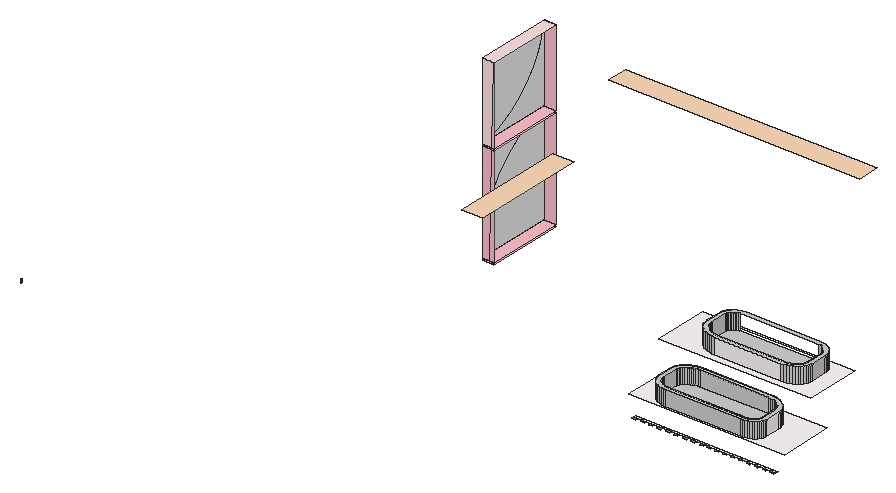
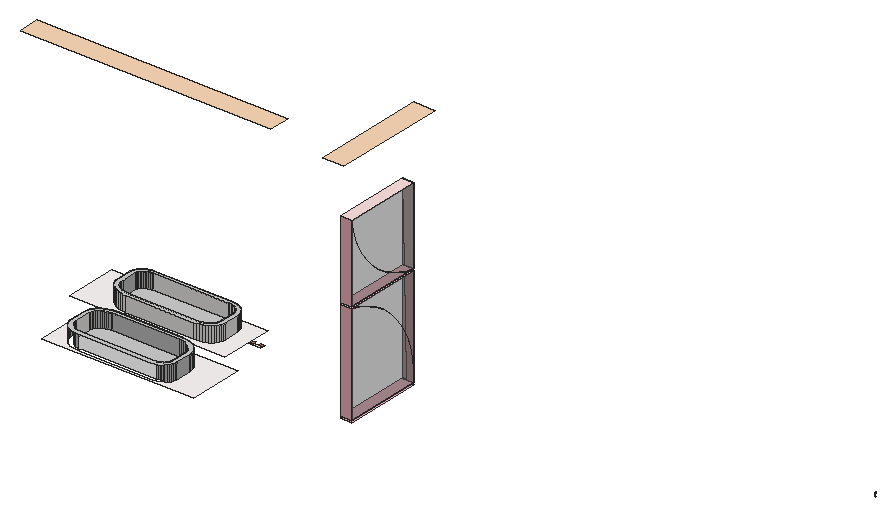
# SketchUp Ruby script. Lengths in inches.
U = 1.inch
M = Sketchup.active_model
def pt(a) = Geom::Point3d.new(a.map { |v| v * U })
def face(e, loops, mat)
  f = e.add_face(loops[0].map { |a| pt(a) })
  loops[1..].each { |l| e.add_face(l.map { |a| pt(a) }).erase! }
  f.material = f.back_material = mat if mat
  f
end
# faces: each face lists its corners as indices into pts; further lists are holes
def faces(e, pts, list, mat = nil) = list.each { |f| face(e, (f[0].is_a?(Array) ? f : [f]).map { |l| l.map { |i| pts[i] } }, mat) }
# xy, xz, yz: faces in a plane at the given z, y or x. An outline is a flat list of corners, or four numbers for a rectangle; further outlines are holes
def ring(l) = l.size == 4 ? [[l[0], l[1]], [l[2], l[1]], [l[2], l[3]], [l[0], l[3]]] : l.each_slice(2).to_a
def flat(e, list, mat, &to3) = list.each { |f| face(e, (f[0].is_a?(Array) ? f : [f]).map { |l| ring(l).map { |u, v| to3.(u, v) } }, mat) }
def xy(e, z, list, mat = nil) = flat(e, list, mat) { |x, y| [x, y, z] }
def xz(e, y, list, mat = nil) = flat(e, list, mat) { |x, z| [x, y, z] }
def yz(e, x, list, mat = nil) = flat(e, list, mat) { |y, z| [x, y, z] }
def lines(e, pts, list) = list.each { |a, b| e.add_line(pt(pts[a]), pt(pts[b])) }
# prism: a flat outline (further loops are holes) pulled along v
def prism(e, loops, v, mat = nil)
  f = face(e, loops, mat); d = Geom::Vector3d.new(v.map { |x| x * U })
  f.pushpull(f.normal.samedirection?(d) ? d.length : -d.length)
end
def box(e, o, s, mat = nil) = prism(e, [[o, [o[0] + s[0], o[1], o[2]], [o[0] + s[0], o[1] + s[1], o[2]], [o[0], o[1] + s[1], o[2]]]], [0, 0, s[2]], mat)
def at(x, y, z, deg = 0) = Geom::Transformation.translation(pt([x, y, z])) * Geom::Transformation.rotation(ORIGIN, Z_AXIS, deg.degrees)
def axes(o, x, y, z) = Geom::Transformation.new([*x, 0, *y, 0, *z, 0, *pt(o).to_a, 1])
def part(name) = M.definitions.add(name)
# library, detail: a bought-in or finely detailed component or shape, given as its bounding box
def library(name, o, s) = part(name).tap { |d| box(d.entities, o, s) }
def detail(e, o, s) = box(e.add_group.entities, o, s)
def put(e, d, t, mat = nil) = e.add_instance(d, t).tap { |i| i.material = mat if mat }
def group(e, t, mat = nil) = e.add_group.tap { |g| g.transformation = t; g.material = mat if mat }.entities
root = M.entities
M.materials.add("Material \#1").color = [140, 140, 140]
M.materials.add("[0006_Pink]").color = [255, 192, 203]
M.materials.add("[0007_MistyRose]").color = [255, 228, 225]
M.materials.add("[0010_Snow]").color = [255, 250, 250]
M.materials.add("[0027_PeachPuff]").color = [255, 218, 185]
M.materials.add("[Carrera Marble]").color = [207, 207, 207]
M.materials.add("[Translucent Glass Gray]").color = [128, 128, 128]
M.materials["[Translucent Glass Gray]"].alpha = 0.5
M.materials.add("[Wood Veneer 02]").color = [190, 128, 91]
xy(root,48.558,[[510.439,237.092,531.02,237.656],[531.507,237.092,551.312,237.656]],"[0010_Snow]")
xy(root,48.558,[[510.439,236.374,511.576,237.092],[512.87,236.374,514.006,237.092],[515.3,236.374,516.437,237.092],[517.731,236.374,518.867,237.092],[520.162,236.374,521.298,237.092],
  [522.592,236.374,523.728,237.092],[525.023,236.374,526.159,237.092],[527.453,236.374,528.59,237.092],[529.884,236.374,531.02,237.092],[531.832,236.374,532.969,237.092],
  [534.125,236.374,535.262,237.092],[536.418,236.374,537.554,237.092],[538.711,236.374,539.847,237.092],[541.004,236.374,542.14,237.092],[543.297,236.374,544.433,237.092],
  [545.59,236.374,546.726,237.092],[547.883,236.374,549.019,237.092],[550.176,236.374,551.312,237.092]],"[Wood Veneer 02]")
xy(root,53.657,[[[508.613,237.656,553.199,252.9375],[518.844,238.177,518.122,238.213,517.413,238.323,516.729,238.503,516.08,238.751,515.479,239.062,514.936,239.432,514.459,239.853,514.057,240.319,513.738,240.822,513.505,241.352,513.364,241.902,513.317,242.461,513.317,246.746,513.365,247.311,513.507,247.866,513.742,248.403,514.065,248.911,514.471,249.382,514.953,249.807,515.502,250.181,516.109,250.495,516.765,250.746,517.456,250.928,518.173,251.039,518.902,251.076,538.502,251.076,539.337,251.033,540.157,250.907,540.949,250.698,541.699,250.412,542.394,250.051,543.023,249.624,543.574,249.137,544.039,248.598,544.408,248.016,544.677,247.402,544.84,246.766,544.895,246.12,544.895,241.774,544.855,241.305,544.737,240.843,544.542,240.398,544.273,239.975,543.936,239.584,543.536,239.23,543.079,238.92,542.575,238.659,542.03,238.451,541.456,238.299,540.86,238.207,540.254,238.177]]],"[0010_Snow]")
xy(root,53.657,[[518.844,239.246,540.254,239.246,540.68,239.267,541.099,239.332,541.503,239.438,541.885,239.585,542.24,239.768,542.561,239.986,542.842,240.235,543.079,240.51,543.268,240.807,543.405,241.12,543.488,241.444,543.516,241.774,543.516,246.12,543.473,246.627,543.345,247.126,543.134,247.607,542.844,248.063,542.48,248.486,542.047,248.868,541.554,249.203,541.009,249.486,540.421,249.711,539.8,249.874,539.157,249.973,538.502,250.006,518.902,250.006,518.353,249.979,517.813,249.895,517.292,249.758,516.799,249.57,516.342,249.333,515.928,249.051,515.565,248.731,515.259,248.376,515.016,247.994,514.839,247.59,514.732,247.171,514.696,246.746,514.696,242.461,514.731,242.042,514.837,241.629,515.012,241.231,515.252,240.853,515.553,240.504,515.911,240.1875,516.319,239.91,516.77,239.677,517.256,239.491,517.77,239.355,518.302,239.273]],"[Carrera Marble]")
xy(root,55.539,[[[500.212,258.9375,543.78,274.779],[514.573,260.868,513.758,260.912,512.957,261.043,512.183,261.259,511.45,261.556,510.77,261.929,510.156,262.372,509.617,262.878,509.163,263.436,508.802,264.039,508.539,264.675,508.38,265.334,508.326,266.005,508.326,270.509,508.365,270.996,508.481,271.474,508.672,271.936,508.934,272.374,509.263,272.779,509.655,273.146,510.1,273.468,510.594,273.739,511.126,273.954,511.6875,274.111,512.269,274.206,512.861,274.238,533.783,274.238,534.488,274.2,535.181,274.087,535.85,273.9,536.483,273.643,537.071,273.321,537.602,272.9375,538.068,272.501,538.46,272.018,538.772,271.497,539,270.947,539.137,270.377,539.184,269.797,539.184,265.356,539.137,264.77,538.998,264.194,538.768,263.638,538.452,263.112,538.056,262.624,537.585,262.182,537.048,261.795,536.455,261.469,535.814,261.209,535.138,261.021,534.438,260.906,533.726,260.868]]],"[0010_Snow]")
xy(root,55.539,[[514.573,261.976,533.726,261.976,534.262,262.005,534.79,262.091,535.299,262.233,535.781,262.429,536.228,262.674,536.632,262.966,536.987,263.298,537.285,263.666,537.523,264.062,537.696,264.481,537.801,264.915,537.836,265.356,537.836,269.797,537.801,270.232,537.698,270.66,537.527,271.073,537.293,271.464,536.998,271.826,536.649,272.154,536.25,272.441,535.809,272.684,535.334,272.876,534.832,273.017,534.312,273.102,533.783,273.13,512.861,273.13,512.445,273.108,512.036,273.041,511.641,272.931,511.267,272.779,510.921,272.589,510.607,272.362,510.332,272.105,510.101,271.82,509.916,271.512,509.782,271.1875,509.701,270.851,509.674,270.509,509.674,266.005,509.716,265.479,509.841,264.962,510.047,264.463,510.33,263.99,510.686,263.552,511.109,263.156,511.591,262.808,512.124,262.516,512.698,262.282,513.305,262.113,513.934,262.01]],"[Carrera Marble]")
xy(root,57.946,[[[518.844,238.177,540.254,238.177,540.86,238.207,541.456,238.299,542.03,238.451,542.575,238.659,543.079,238.92,543.536,239.23,543.936,239.584,544.273,239.975,544.542,240.398,544.737,240.843,544.855,241.305,544.895,241.774,544.895,246.12,544.84,246.766,544.677,247.402,544.408,248.016,544.039,248.598,543.574,249.137,543.023,249.624,542.394,250.051,541.699,250.412,540.949,250.698,540.157,250.907,539.337,251.033,538.502,251.076,518.902,251.076,518.173,251.039,517.456,250.928,516.765,250.746,516.109,250.495,515.502,250.181,514.953,249.807,514.471,249.382,514.065,248.911,513.742,248.403,513.507,247.866,513.365,247.311,513.317,246.746,513.317,242.461,513.364,241.902,513.505,241.352,513.738,240.822,514.057,240.319,514.459,239.853,514.936,239.432,515.479,239.062,516.08,238.751,516.729,238.503,517.413,238.323,518.122,238.213],[518.844,239.246,518.302,239.273,517.77,239.355,517.256,239.491,516.77,239.677,516.319,239.91,515.911,240.1875,515.553,240.504,515.252,240.853,515.012,241.231,514.837,241.629,514.731,242.042,514.696,242.461,514.696,246.746,514.732,247.171,514.839,247.59,515.016,247.994,515.259,248.376,515.565,248.731,515.928,249.051,516.342,249.333,516.799,249.57,517.292,249.758,517.813,249.895,518.353,249.979,518.902,250.006,538.502,250.006,539.157,249.973,539.8,249.874,540.421,249.711,541.009,249.486,541.554,249.203,542.047,248.868,542.48,248.486,542.844,248.063,543.134,247.607,543.345,247.126,543.473,246.627,543.516,246.12,543.516,241.774,543.488,241.444,543.405,241.12,543.268,240.807,543.079,240.51,542.842,240.235,542.561,239.986,542.24,239.768,541.885,239.585,541.503,239.438,541.099,239.332,540.68,239.267,540.254,239.246]]],"[Carrera Marble]")
xy(root,59.978,[[[514.573,260.868,533.726,260.868,534.438,260.906,535.138,261.021,535.814,261.209,536.455,261.469,537.048,261.795,537.585,262.182,538.056,262.624,538.452,263.112,538.768,263.638,538.998,264.194,539.137,264.77,539.184,265.356,539.184,269.797,539.137,270.377,539,270.947,538.772,271.497,538.46,272.018,538.068,272.501,537.602,272.9375,537.071,273.321,536.483,273.643,535.85,273.9,535.181,274.087,534.488,274.2,533.783,274.238,512.861,274.238,512.269,274.206,511.6875,274.111,511.126,273.954,510.594,273.739,510.1,273.468,509.655,273.146,509.263,272.779,508.934,272.374,508.672,271.936,508.481,271.474,508.365,270.996,508.326,270.509,508.326,266.005,508.38,265.334,508.539,264.675,508.802,264.039,509.163,263.436,509.617,262.878,510.156,262.372,510.77,261.929,511.45,261.556,512.183,261.259,512.957,261.043,513.758,260.912],[514.573,261.976,513.934,262.01,513.305,262.113,512.698,262.282,512.124,262.516,511.591,262.808,511.109,263.156,510.686,263.552,510.33,263.99,510.047,264.463,509.841,264.962,509.716,265.479,509.674,266.005,509.674,270.509,509.701,270.851,509.782,271.1875,509.916,271.512,510.101,271.82,510.332,272.105,510.607,272.362,510.921,272.589,511.267,272.779,511.641,272.931,512.036,273.041,512.445,273.108,512.861,273.13,533.783,273.13,534.312,273.102,534.832,273.017,535.334,272.876,535.809,272.684,536.25,272.441,536.649,272.154,536.998,271.826,537.293,271.464,537.527,271.073,537.698,270.66,537.801,270.232,537.836,269.797,537.836,265.356,537.801,264.915,537.696,264.481,537.523,264.062,537.285,263.666,536.987,263.298,536.632,262.966,536.228,262.674,535.781,262.429,535.299,262.233,534.79,262.091,534.262,262.005,533.726,261.976]]],"[Carrera Marble]")
xy(root,63.875,[[456.0625,250.71,459.4375,272.96]],"[0006_Pink]")
xy(root,64.375,[[456.0625,250.71,459.4375,272.96]],"[0006_Pink]")
xy(root,93.125,[[456.0625,250.71,459.4375,272.96]],"[0006_Pink]")
xy(root,93.625,[[456.0625,250.71,459.4375,272.96]],"[0006_Pink]")
xy(root,105.5625,[[484.5625,207.773,490.5625,240.508]],"[0027_PeachPuff]")
xy(root,115.8125,[[456.0625,250.71,459.4375,272.96]],"[0007_MistyRose]")
xy(root,121.1875,[[490.5625,252.9375,562.5625,258.9375]],"[0027_PeachPuff]")
xz(root,238.177,[[518.844,53.657,540.254,57.946]],"[Carrera Marble]")
xz(root,239.246,[[518.844,53.657,540.254,57.946]],"[0010_Snow]")
xz(root,250.006,[[518.902,53.657,538.502,57.946]],"[Carrera Marble]")
xz(root,250.71,[[458.133,63.875,459.4375,63.875,459.4375,64.375,458.146,64.375],[456.0625,64.375,458.146,64.375,458.868,93.125,456.0625,93.125],[458.146,64.375,459.4375,64.375,459.4375,93.125,458.868,93.125],[458.868,93.125,459.4375,93.125,459.4375,93.625,458.88,93.625],[458.88,93.625,459.4375,93.625,459.4375,115.8125]],"[0006_Pink]")
xz(root,250.71,[[456.0625,93.625,458.88,93.625,459.4375,115.8125,456.0625,115.8125]],"[0007_MistyRose]")
xz(root,251.076,[[518.902,53.657,538.502,57.946]],"[0010_Snow]")
xz(root,260.868,[[514.573,55.539,533.726,59.978]],"[0010_Snow]")
xz(root,261.976,[[514.573,55.539,533.726,59.978]],"[Carrera Marble]")
xz(root,272.96,[[456.0625,64.375,459.4375,93.125],[456.0625,93.625,459.4375,115.8125]],"[0006_Pink]")
yz(root,362.6875,[[201.873,46.505,201.932,46.557,201.905,46.528],[201.932,46.557,201.965,46.631,201.952,46.591],[201.932,46.557,201.97,47.032,201.965,46.631],[201.965,46.631,201.97,47.032,201.97,46.674],[201.985,47.073,202.044,47.139,201.991,47.079],
  [201.991,47.079,202.044,47.139,202.019,47.107]],"Material \#1")
yz(root,362.688,[[201.798,47.076,201.735,47.085,201.738,47.094],[201.798,47.076,201.738,47.094,201.798,47.086],[201.798,47.076,201.798,47.086,201.86,47.085],[201.735,47.085,201.677,47.111,201.681,47.12],[201.735,47.085,201.681,47.12,201.738,47.094],
  [201.86,47.085,201.798,47.086,201.858,47.094],[201.86,47.085,201.858,47.094,201.919,47.111],[201.858,47.094,201.914,47.12,201.919,47.111],[201.677,47.111,201.627,47.153,201.633,47.16],[201.677,47.111,201.633,47.16,201.681,47.12],
  [201.919,47.111,201.914,47.12,201.969,47.153],[201.914,47.12,201.962,47.16,201.969,47.153],[201.627,47.153,201.588,47.208,201.596,47.213],[201.627,47.153,201.596,47.213,201.633,47.16],[201.969,47.153,201.962,47.16,202.007,47.208],
  [201.962,47.16,201.999,47.213,202.007,47.208],[201.588,47.208,201.564,47.271,201.573,47.274],[201.588,47.208,201.573,47.274,201.596,47.213],[202.007,47.208,201.999,47.213,202.031,47.271],[201.999,47.213,202.023,47.274,202.031,47.271],
  [201.564,47.271,201.556,47.34,201.565,47.34],[201.564,47.271,201.565,47.34,201.573,47.274],[202.031,47.271,202.023,47.274,202.04,47.34],[202.023,47.274,202.031,47.34,202.04,47.34],[201.556,47.34,201.564,47.408,201.573,47.405],
  [201.556,47.34,201.573,47.405,201.565,47.34],[202.031,47.34,202.023,47.405,202.031,47.408],[202.031,47.34,202.031,47.408,202.04,47.34],[201.573,47.405,201.564,47.408,201.596,47.466],[202.023,47.405,201.999,47.466,202.007,47.471],
  [202.023,47.405,202.007,47.471,202.031,47.408],[201.564,47.408,201.588,47.471,201.596,47.466],[201.596,47.466,201.588,47.471,201.633,47.519],[201.999,47.466,201.962,47.519,201.969,47.526],[201.999,47.466,201.969,47.526,202.007,47.471],
  [201.588,47.471,201.627,47.526,201.633,47.519],[201.633,47.519,201.627,47.526,201.681,47.559],[201.962,47.519,201.914,47.559,201.919,47.568],[201.962,47.519,201.919,47.568,201.969,47.526],[201.627,47.526,201.677,47.568,201.681,47.559],
  [201.681,47.559,201.677,47.568,201.738,47.585],[201.914,47.559,201.858,47.585,201.86,47.594],[201.914,47.559,201.86,47.594,201.919,47.568],[201.677,47.568,201.735,47.594,201.738,47.585],[201.738,47.585,201.735,47.594,201.798,47.593],
  [201.858,47.585,201.798,47.593,201.798,47.603],[201.858,47.585,201.798,47.603,201.86,47.594],[201.798,47.593,201.735,47.594,201.798,47.603]],"Material \#1")
yz(root,456.0625,[[250.71,64.375,250.71,93.125,272.96,93.125,269.773,92.276,266.708,91.056,263.808,89.482,261.116,87.577,258.667,85.366,256.497,82.881,254.636,80.157,253.11,77.233,251.941,74.148,251.145,70.947,250.733,67.674],[250.71,64.375,250.733,67.674,251.145,70.947,251.941,74.148,253.11,77.233,254.636,80.157,256.497,82.881,258.667,85.366,261.116,87.577,263.808,89.482,266.708,91.056,269.773,92.276,272.96,93.125,272.96,64.375],[250.71,93.625,250.71,115.8125,272.96,115.8125,272.415,113.058,271.577,110.378,270.456,107.804,269.065,105.364,267.421,103.088,265.542,101.001,263.45,99.128,261.17,97.49,258.726,96.107,256.149,94.993,253.466,94.163],[250.71,93.625,253.466,94.163,256.149,94.993,258.726,96.107,261.17,97.49,263.45,99.128,265.542,101.001,267.421,103.088,269.065,105.364,270.456,107.804,271.577,110.378,272.415,113.058,272.96,115.8125,272.96,93.625]],"[Translucent Glass Gray]")
yz(root,508.326,[[266.005,55.539,270.509,59.978]],"[Carrera Marble]")
yz(root,509.674,[[266.005,55.539,270.509,59.978]],"[Carrera Marble]")
yz(root,513.317,[[242.461,53.657,246.746,57.946]],"[0010_Snow]")
yz(root,514.696,[[242.461,53.657,246.746,57.946]],"[Carrera Marble]")
yz(root,537.836,[[265.356,55.539,269.797,59.978]],"[0010_Snow]")
yz(root,539.184,[[265.356,55.539,269.797,59.978]],"[Carrera Marble]")
yz(root,543.516,[[241.774,53.657,246.12,57.946]],"[Carrera Marble]")
yz(root,544.895,[[241.774,53.657,246.12,57.946]],"[0010_Snow]")
p = [[517.413,238.323,53.657],[518.122,238.213,53.657],[518.122,238.213,57.946],[517.413,238.323,57.946],[518.844,238.177,53.657],[518.844,238.177,57.946],
  [540.254,238.177,53.657],[540.86,238.207,53.657],[540.86,238.207,57.946],[540.254,238.177,57.946],[541.456,238.299,53.657],[541.456,238.299,57.946],
  [516.729,238.503,53.657],[516.729,238.503,57.946],[542.03,238.451,53.657],[542.03,238.451,57.946],[516.08,238.751,53.657],[516.08,238.751,57.946],
  [542.575,238.659,53.657],[542.575,238.659,57.946],[543.079,238.92,53.657],[543.079,238.92,57.946],[515.479,239.062,53.657],[515.479,239.062,57.946],
  [543.536,239.23,53.657],[543.536,239.23,57.946],[514.936,239.432,53.657],[514.936,239.432,57.946],[518.844,239.246,53.657],[518.302,239.273,53.657],
  [518.302,239.273,57.946],[518.844,239.246,57.946],[540.68,239.267,53.657],[540.254,239.246,53.657],[540.254,239.246,57.946],[540.68,239.267,57.946],
  [543.936,239.584,53.657],[543.936,239.584,57.946],[517.77,239.355,53.657],[517.77,239.355,57.946],[541.099,239.332,53.657],[541.099,239.332,57.946],
  [541.503,239.438,53.657],[541.503,239.438,57.946],[514.459,239.853,53.657],[514.459,239.853,57.946],[517.256,239.491,53.657],[517.256,239.491,57.946],
  [541.885,239.585,53.657],[541.885,239.585,57.946],[516.77,239.677,53.657],[516.77,239.677,57.946],[542.24,239.768,53.657],[542.24,239.768,57.946],
  [544.273,239.975,53.657],[544.273,239.975,57.946],[516.319,239.91,53.657],[516.319,239.91,57.946],[542.561,239.986,53.657],[542.561,239.986,57.946],
  [514.057,240.319,53.657],[514.057,240.319,57.946],[515.911,240.1875,53.657],[515.911,240.1875,57.946],[542.842,240.235,53.657],[542.842,240.235,57.946],
  [544.542,240.398,53.657],[544.542,240.398,57.946],[515.553,240.504,53.657],[515.553,240.504,57.946],[543.079,240.51,53.657],[543.079,240.51,57.946],
  [513.738,240.822,53.657],[513.738,240.822,57.946],[544.737,240.843,53.657],[544.737,240.843,57.946],[515.252,240.853,53.657],[515.252,240.853,57.946],
  [543.268,240.807,53.657],[543.268,240.807,57.946],[513.505,241.352,53.657],[513.505,241.352,57.946],[543.405,241.12,53.657],[543.405,241.12,57.946],
  [544.855,241.305,53.657],[544.855,241.305,57.946],[515.012,241.231,53.657],[515.012,241.231,57.946],[543.488,241.444,53.657],[543.488,241.444,57.946],
  [514.837,241.629,53.657],[514.837,241.629,57.946],[544.895,241.774,53.657],[544.895,241.774,57.946],[513.364,241.902,53.657],[513.364,241.902,57.946],
  [543.516,241.774,53.657],[543.516,241.774,57.946],[514.731,242.042,53.657],[514.731,242.042,57.946],[513.317,242.461,53.657],[513.317,242.461,57.946],
  [514.696,242.461,53.657],[514.696,242.461,57.946],[543.473,246.627,53.657],[543.516,246.12,53.657],[543.516,246.12,57.946],[543.473,246.627,57.946],
  [544.895,246.12,53.657],[544.84,246.766,53.657],[544.84,246.766,57.946],[544.895,246.12,57.946],[543.345,247.126,53.657],[543.345,247.126,57.946],
  [513.365,247.311,53.657],[513.317,246.746,53.657],[513.317,246.746,57.946],[513.365,247.311,57.946],[514.696,246.746,53.657],[514.732,247.171,53.657],
  [514.732,247.171,57.946],[514.696,246.746,57.946],[544.677,247.402,53.657],[544.677,247.402,57.946],[543.134,247.607,53.657],[543.134,247.607,57.946],
  [514.839,247.59,53.657],[514.839,247.59,57.946],[513.507,247.866,53.657],[513.507,247.866,57.946],[544.408,248.016,53.657],[544.408,248.016,57.946],
  [515.016,247.994,53.657],[515.016,247.994,57.946],[542.844,248.063,53.657],[542.844,248.063,57.946],[513.742,248.403,53.657],[513.742,248.403,57.946],
  [515.259,248.376,53.657],[515.259,248.376,57.946],[544.039,248.598,53.657],[544.039,248.598,57.946],[542.48,248.486,53.657],[542.48,248.486,57.946],
  [514.065,248.911,53.657],[514.065,248.911,57.946],[515.565,248.731,53.657],[515.565,248.731,57.946],[542.047,248.868,53.657],[542.047,248.868,57.946],
  [543.574,249.137,53.657],[543.574,249.137,57.946],[515.928,249.051,53.657],[515.928,249.051,57.946],[514.471,249.382,53.657],[514.471,249.382,57.946],
  [541.554,249.203,53.657],[541.554,249.203,57.946],[516.342,249.333,53.657],[516.342,249.333,57.946],[543.023,249.624,53.657],[543.023,249.624,57.946],
  [541.009,249.486,53.657],[541.009,249.486,57.946],[516.799,249.57,53.657],[516.799,249.57,57.946],[514.953,249.807,53.657],[514.953,249.807,57.946],
  [540.421,249.711,53.657],[540.421,249.711,57.946],[517.292,249.758,53.657],[517.292,249.758,57.946],[542.394,250.051,53.657],[542.394,250.051,57.946],
  [539.8,249.874,53.657],[539.8,249.874,57.946],[515.502,250.181,53.657],[515.502,250.181,57.946],[517.813,249.895,53.657],[517.813,249.895,57.946],
  [518.353,249.979,53.657],[518.353,249.979,57.946],[539.157,249.973,53.657],[539.157,249.973,57.946],[518.902,250.006,53.657],[518.902,250.006,57.946],
  [538.502,250.006,53.657],[538.502,250.006,57.946],[541.699,250.412,53.657],[541.699,250.412,57.946],[516.109,250.495,53.657],[516.109,250.495,57.946],
  [540.949,250.698,53.657],[540.949,250.698,57.946],[516.765,250.746,53.657],[516.765,250.746,57.946],[517.456,250.928,53.657],[517.456,250.928,57.946],
  [540.157,250.907,53.657],[540.157,250.907,57.946],[518.173,251.039,53.657],[518.173,251.039,57.946],[539.337,251.033,53.657],[539.337,251.033,57.946],
  [518.902,251.076,53.657],[518.902,251.076,57.946],[538.502,251.076,53.657],[538.502,251.076,57.946],[512.957,261.043,55.539],[513.758,260.912,55.539],
  [513.758,260.912,59.978],[512.957,261.043,59.978],[514.573,260.868,55.539],[514.573,260.868,59.978],[533.726,260.868,55.539],[534.438,260.906,55.539],
  [534.438,260.906,59.978],[533.726,260.868,59.978],[535.138,261.021,55.539],[535.138,261.021,59.978],[512.183,261.259,55.539],[512.183,261.259,59.978],
  [535.814,261.209,55.539],[535.814,261.209,59.978],[536.455,261.469,55.539],[536.455,261.469,59.978],[511.45,261.556,55.539],[511.45,261.556,59.978],
  [537.048,261.795,55.539],[537.048,261.795,59.978],[510.77,261.929,55.539],[510.77,261.929,59.978],[537.585,262.182,55.539],[537.585,262.182,59.978],
  [510.156,262.372,55.539],[510.156,262.372,59.978],[513.934,262.01,55.539],[513.305,262.113,55.539],[513.305,262.113,59.978],[513.934,262.01,59.978],
  [514.573,261.976,55.539],[514.573,261.976,59.978],[534.262,262.005,55.539],[533.726,261.976,55.539],[533.726,261.976,59.978],[534.262,262.005,59.978],
  [534.79,262.091,55.539],[534.79,262.091,59.978],[512.698,262.282,55.539],[512.698,262.282,59.978],[535.299,262.233,55.539],[535.299,262.233,59.978],
  [535.781,262.429,55.539],[535.781,262.429,59.978],[538.056,262.624,55.539],[538.056,262.624,59.978],[512.124,262.516,55.539],[512.124,262.516,59.978],
  [509.617,262.878,55.539],[509.617,262.878,59.978],[536.228,262.674,55.539],[536.228,262.674,59.978],[511.591,262.808,55.539],[511.591,262.808,59.978],
  [538.452,263.112,55.539],[538.452,263.112,59.978],[536.632,262.966,55.539],[536.632,262.966,59.978],[511.109,263.156,55.539],[511.109,263.156,59.978],
  [509.163,263.436,55.539],[509.163,263.436,59.978],[536.987,263.298,55.539],[536.987,263.298,59.978],[538.768,263.638,55.539],[538.768,263.638,59.978],
  [510.686,263.552,55.539],[510.686,263.552,59.978],[537.285,263.666,55.539],[537.285,263.666,59.978],[508.802,264.039,55.539],[508.802,264.039,59.978],
  [510.33,263.99,55.539],[510.33,263.99,59.978],[538.998,264.194,55.539],[538.998,264.194,59.978],[537.523,264.062,55.539],[537.523,264.062,59.978],
  [508.539,264.675,55.539],[508.539,264.675,59.978],[510.047,264.463,55.539],[510.047,264.463,59.978],[537.696,264.481,55.539],[537.696,264.481,59.978],
  [539.137,264.77,55.539],[539.137,264.77,59.978],[509.841,264.962,55.539],[509.841,264.962,59.978],[537.801,264.915,55.539],[537.801,264.915,59.978],
  [508.38,265.334,55.539],[508.38,265.334,59.978],[539.184,265.356,55.539],[539.184,265.356,59.978],[537.836,265.356,55.539],[537.836,265.356,59.978],
  [509.716,265.479,55.539],[509.716,265.479,59.978],[508.326,266.005,55.539],[508.326,266.005,59.978],[509.674,266.005,55.539],[509.674,266.005,59.978],
  [537.801,270.232,55.539],[537.836,269.797,55.539],[537.836,269.797,59.978],[537.801,270.232,59.978],[539.184,269.797,55.539],[539.137,270.377,55.539],
  [539.137,270.377,59.978],[539.184,269.797,59.978],[537.698,270.66,55.539],[537.698,270.66,59.978],[539,270.947,55.539],[539,270.947,59.978],
  [508.365,270.996,55.539],[508.326,270.509,55.539],[508.326,270.509,59.978],[508.365,270.996,59.978],[509.674,270.509,55.539],[509.701,270.851,55.539],
  [509.701,270.851,59.978],[509.674,270.509,59.978],[537.527,271.073,55.539],[537.527,271.073,59.978],[509.782,271.1875,55.539],[509.782,271.1875,59.978],
  [538.772,271.497,55.539],[538.772,271.497,59.978],[508.481,271.474,55.539],[508.481,271.474,59.978],[537.293,271.464,55.539],[537.293,271.464,59.978],
  [509.916,271.512,55.539],[509.916,271.512,59.978],[508.672,271.936,55.539],[508.672,271.936,59.978],[510.101,271.82,55.539],[510.101,271.82,59.978],
  [536.998,271.826,55.539],[536.998,271.826,59.978],[538.46,272.018,55.539],[538.46,272.018,59.978],[510.332,272.105,55.539],[510.332,272.105,59.978],
  [536.649,272.154,55.539],[536.649,272.154,59.978],[508.934,272.374,55.539],[508.934,272.374,59.978],[538.068,272.501,55.539],[538.068,272.501,59.978],
  [510.607,272.362,55.539],[510.607,272.362,59.978],[536.25,272.441,55.539],[536.25,272.441,59.978],[509.263,272.779,55.539],[509.263,272.779,59.978],
  [510.921,272.589,55.539],[510.921,272.589,59.978],[535.809,272.684,55.539],[535.809,272.684,59.978],[537.602,272.9375,55.539],[537.602,272.9375,59.978],
  [511.267,272.779,55.539],[511.267,272.779,59.978],[535.334,272.876,55.539],[535.334,272.876,59.978],[509.655,273.146,55.539],[509.655,273.146,59.978],
  [511.641,272.931,55.539],[511.641,272.931,59.978],[512.036,273.041,55.539],[512.036,273.041,59.978],[534.832,273.017,55.539],[534.832,273.017,59.978]]
faces(root,p,[[0,1,2,3],[1,4,5,2],[6,7,8,9],[7,10,11,8],[12,0,3,13],[10,14,15,11],[16,12,13,17],[14,18,19,15],
  [18,20,21,19],[22,16,17,23],[20,24,25,21],[26,22,23,27],[32,33,34,35],[24,36,37,25],[40,32,35,41],[42,40,41,43],
  [44,26,27,45],[48,42,43,49],[52,48,49,53],[36,54,55,37],[58,52,53,59],[60,44,45,61],[64,58,59,65],[54,66,67,55],
  [70,64,65,71],[72,60,61,73],[66,74,75,67],[78,70,71,79],[80,72,73,81],[82,78,79,83],[74,84,85,75],[88,82,83,89],
  [84,92,93,85],[94,80,81,95],[96,88,89,97],[100,94,95,101],[104,105,106,107],[112,104,107,113],[118,119,120,121],[124,112,113,125],
  [119,126,127,120],[126,132,133,127],[134,124,125,135],[132,138,139,133],[142,134,135,143],[138,146,147,139],[148,142,143,149],[146,152,153,147],
  [156,148,149,157],[152,158,159,153],[162,156,157,163],[158,164,165,159],[168,162,163,169],[164,170,171,165],[174,168,169,175],[170,178,179,171],
  [178,180,181,179],[182,174,175,183],[180,184,185,181],[186,182,183,187],[208,209,210,211],[209,212,213,210],[214,215,216,217],[215,218,219,216],
  [220,208,211,221],[218,222,223,219],[222,224,225,223],[226,220,221,227],[224,228,229,225],[230,226,227,231],[228,232,233,229],[234,230,231,235],
  [236,237,238,239],[240,236,239,241],[242,243,244,245],[246,242,245,247],[237,248,249,238],[250,246,247,251],[252,250,251,253],[232,254,255,233],
  [248,256,257,249],[258,234,235,259],[260,252,253,261],[256,262,263,257],[254,264,265,255],[266,260,261,267],[262,268,269,263],[270,258,259,271],
  [272,266,267,273],[264,274,275,265],[268,276,277,269],[278,272,273,279],[280,270,271,281],[276,282,283,277],[274,284,285,275],[286,278,279,287],
  [288,280,281,289],[282,290,291,283],[292,286,287,293],[284,294,295,285],[290,296,297,291],[298,292,293,299],[300,288,289,301],[294,302,303,295],
  [304,298,299,305],[296,306,307,297],[308,300,301,309],[306,310,311,307],[312,313,314,315],[316,317,318,319],[320,312,315,321],[317,322,323,318],
  [324,325,326,327],[328,329,330,331],[332,320,321,333],[329,334,335,330],[322,336,337,323],[338,324,327,339],[340,332,333,341],[334,342,343,335],
  [344,338,339,345],[342,346,347,343],[348,340,341,349],[336,350,351,337],[346,352,353,347],[354,348,349,355],[356,344,345,357],[350,358,359,351],
  [352,360,361,353],[362,354,355,363],[364,356,357,365],[360,366,367,361],[368,362,363,369],[358,370,371,359],[366,372,373,367],[374,368,369,375],
  [376,364,365,377],[372,378,379,373],[378,380,381,379],[382,374,375,383]],"[Carrera Marble]")
faces(root,p,[[28,29,30,31],[29,38,39,30],[38,46,47,39],[46,50,51,47],[50,56,57,51],[56,62,63,57],[62,68,69,63],[68,76,77,69],
  [76,86,87,77],[86,90,91,87],[90,98,99,91],[98,102,103,99],[108,109,110,111],[114,115,116,117],[109,122,123,110],[128,114,117,129],
  [122,130,131,123],[136,128,129,137],[130,140,141,131],[144,136,137,145],[140,150,151,141],[154,144,145,155],[150,160,161,151],[166,154,155,167],
  [160,172,173,161],[176,166,167,177],[172,188,189,173],[190,176,177,191],[188,192,193,189],[194,190,191,195],[196,194,195,197],[192,198,199,193],
  [200,196,197,201],[198,202,203,199],[204,200,201,205],[202,206,207,203]],"[0010_Snow]")
